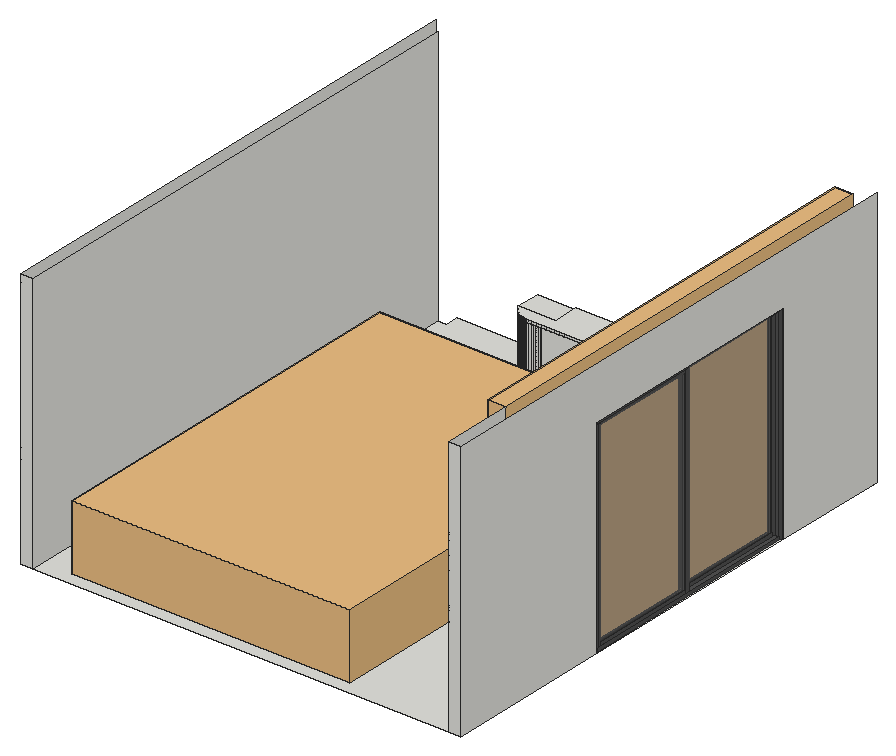
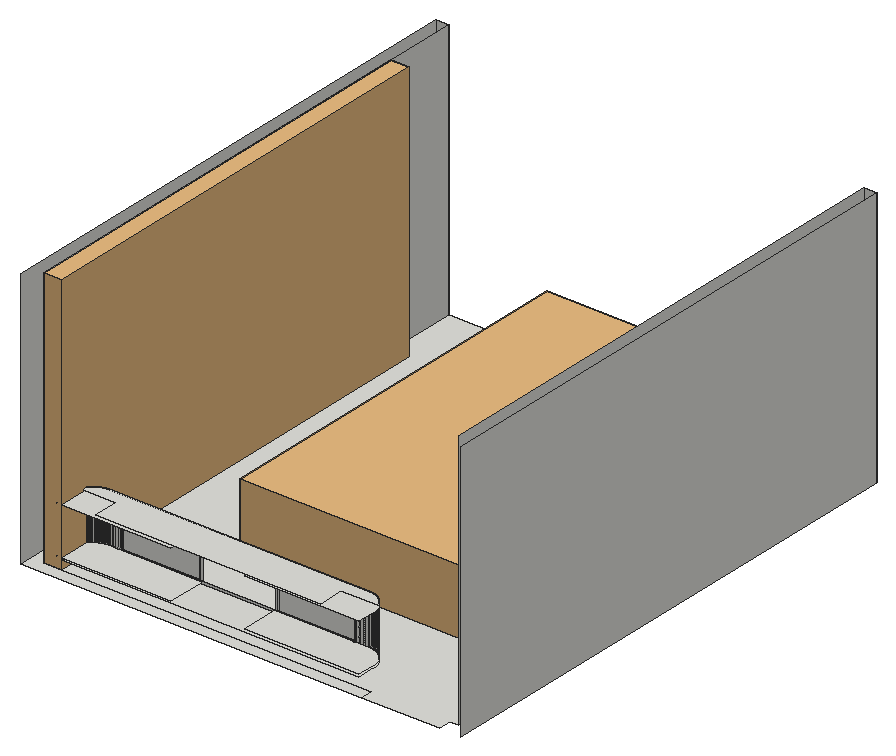
# SketchUp Ruby script. Lengths in inches.
U = 1.inch
M = Sketchup.active_model
def pt(a) = Geom::Point3d.new(a.map { |v| v * U })
def face(e, loops, mat)
  f = e.add_face(loops[0].map { |a| pt(a) })
  loops[1..].each { |l| e.add_face(l.map { |a| pt(a) }).erase! }
  f.material = f.back_material = mat if mat
  f
end
# faces: each face lists its corners as indices into pts; further lists are holes
def faces(e, pts, list, mat = nil) = list.each { |f| face(e, (f[0].is_a?(Array) ? f : [f]).map { |l| l.map { |i| pts[i] } }, mat) }
# xy, xz, yz: faces in a plane at the given z, y or x. An outline is a flat list of corners, or four numbers for a rectangle; further outlines are holes
def ring(l) = l.size == 4 ? [[l[0], l[1]], [l[2], l[1]], [l[2], l[3]], [l[0], l[3]]] : l.each_slice(2).to_a
def flat(e, list, mat, &to3) = list.each { |f| face(e, (f[0].is_a?(Array) ? f : [f]).map { |l| ring(l).map { |u, v| to3.(u, v) } }, mat) }
def xy(e, z, list, mat = nil) = flat(e, list, mat) { |x, y| [x, y, z] }
def xz(e, y, list, mat = nil) = flat(e, list, mat) { |x, z| [x, y, z] }
def yz(e, x, list, mat = nil) = flat(e, list, mat) { |y, z| [x, y, z] }
def lines(e, pts, list) = list.each { |a, b| e.add_line(pt(pts[a]), pt(pts[b])) }
# prism: a flat outline (further loops are holes) pulled along v
def prism(e, loops, v, mat = nil)
  f = face(e, loops, mat); d = Geom::Vector3d.new(v.map { |x| x * U })
  f.pushpull(f.normal.samedirection?(d) ? d.length : -d.length)
end
def box(e, o, s, mat = nil) = prism(e, [[o, [o[0] + s[0], o[1], o[2]], [o[0] + s[0], o[1] + s[1], o[2]], [o[0], o[1] + s[1], o[2]]]], [0, 0, s[2]], mat)
def at(x, y, z, deg = 0) = Geom::Transformation.translation(pt([x, y, z])) * Geom::Transformation.rotation(ORIGIN, Z_AXIS, deg.degrees)
def axes(o, x, y, z) = Geom::Transformation.new([*x, 0, *y, 0, *z, 0, *pt(o).to_a, 1])
def part(name) = M.definitions.add(name)
# library, detail: a bought-in or finely detailed component or shape, given as its bounding box
def library(name, o, s) = part(name).tap { |d| box(d.entities, o, s) }
def detail(e, o, s) = box(e.add_group.entities, o, s)
def put(e, d, t, mat = nil) = e.add_instance(d, t).tap { |i| i.material = mat if mat }
def group(e, t, mat = nil) = e.add_group.tap { |g| g.transformation = t; g.material = mat if mat }.entities
root = M.entities
M.materials.add("[0049_Beige]").color = [245, 245, 220]
M.materials.add("[0135_DarkGray]").color = [81, 81, 81]
M.materials.add("[0136_Charcoal]").color = [35, 35, 35]
M.materials.add("[Aluminum]").color = [179, 179, 179]
M.materials.add("[Translucent Glass Gray]").color = [128, 128, 128]
M.materials["[Translucent Glass Gray]"].alpha = 0.15
c1 = library("Sofa+Set+3+(1)",[-143.38,0,0],[143.38,111.7,30.22])
c2 = part("PENTEK_RP Fineline 50S_Sliding_DoorCase_E1")
box(c2.entities,[0,0,0],[1.51,3.66,99.27],"[0135_DarkGray]")
c3 = part("PENTEK_RP Fineline 50S_SlidingDooe_Case_E2")
box(c3.entities,[0,0,0],[96.25,3.66,1.51],"[0135_DarkGray]")
c4 = part("pentek_RP Fineline 50S_SlidingDoor_Case")
put(c4.entities,c2,at(97.76,0,0))
put(c4.entities,c3,at(1.51,0,0))
put(c4.entities,c2,at(0,0,0))
put(c4.entities,c3,at(1.51,0,97.76))
c5 = part("PENTEK_RP Fineline 50S_SlidingDoor_Glass")
box(c5.entities,[0,0,0],[46.58,0.16,94.39],"[Translucent Glass Gray]")
c6 = part("PENTEK_RP Fineline 50S_SlidingDoor_GlazingBead")
box(c6.entities,[0,0,0],[45.47,0.59,0.56],"[0135_DarkGray]")
c7 = part("PENTEK_RP Fineline 50S_SlidingDoor_GlazingBead_2")
box(c7.entities,[0,0,0],[0.56,0.59,94.39],"[0135_DarkGray]")
c8 = part("PENTEK_RP Fineline 50S_SlidingDoor_Leaf_E1")
xy(c8.entities,0,[[0,0,0.93,1.97],[0.93,1.57,1.49,1.97]],"[0135_DarkGray]")
xy(c8.entities,96.25,[[0,0,0.93,0,0.93,1.57,1.49,1.57,1.49,1.97,0,1.97]],"[0135_DarkGray]")
xz(c8.entities,0,[[0,0,0.93,96.25]],"[0135_DarkGray]")
xz(c8.entities,1.57,[[0.93,0,1.49,95.32],[0.93,95.32,1.49,96.25]],"[0135_DarkGray]")
xz(c8.entities,1.97,[[0,0,1.49,96.25]],"[0135_DarkGray]")
yz(c8.entities,0,[[0,0,1.97,96.25]],"[0135_DarkGray]")
yz(c8.entities,0.93,[[0,0,1.57,0.93],[0,0.93,1.57,95.32],[0,95.32,1.57,96.25]],"[0135_DarkGray]")
yz(c8.entities,1.49,[[1.57,0,1.97,95.32],[1.57,95.32,1.97,96.25]],"[0135_DarkGray]")
c9 = part("PENTEK_RP Fineline 50S_SlidingDoor_Leaf_E2")
xy(c9.entities,0,[[0,0,0,1.57,0.56,1.57,0.56,1.97,46.02,1.97,46.02,1.57,46.58,1.57,46.58,0]],"[0135_DarkGray]")
xy(c9.entities,0.93,[[0,0,46.58,1.57]],"[0135_DarkGray]")
xy(c9.entities,1.49,[[0.56,1.57,46.02,1.97]],"[0135_DarkGray]")
xz(c9.entities,0,[[0,0,46.58,0.93]],"[0135_DarkGray]")
xz(c9.entities,1.57,[[0,0,0.56,0.93],[46.02,0,46.58,0.93],[0.56,0.93,46.02,1.49]],"[0135_DarkGray]")
xz(c9.entities,1.97,[[0.56,0,46.02,1.49]],"[0135_DarkGray]")
yz(c9.entities,0,[[0,0,1.57,0.93]],"[0135_DarkGray]")
yz(c9.entities,0.56,[[1.57,0,1.97,0.93],[1.57,0.93,1.97,1.49]],"[0135_DarkGray]")
yz(c9.entities,46.02,[[1.57,0,1.97,0.93],[1.57,0.93,1.97,1.49]],"[0135_DarkGray]")
yz(c9.entities,46.58,[[0,0,1.57,0.93]],"[0135_DarkGray]")
c10 = part("PENTEK_RP Fineline 50S_SlidingDoor_Leaf2")
put(c10.entities,c5,at(1.49,1.42,0.93))
put(c10.entities,c6,at(1.49,0,94.77))
put(c10.entities,c7,at(46.96,0,0.93))
put(c10.entities,c5,at(1.49,0.59,0.93))
put(c10.entities,c7,at(0.93,0,0.93))
put(c10.entities,c8,at(0,0,0))
put(c10.entities,c8,axes([48.44,0,0],[-1,0,0],[0,1,0],[0,0,1]))
put(c10.entities,c6,at(1.49,0,0.93))
put(c10.entities,c9,axes([0.93,0,96.25],[1,0,0],[0,1,0],[0,0,-1]))
put(c10.entities,c9,at(0.93,0,0))
c11 = part("PENTEK_RP Fineline S_SlidingDoor_Leaf1")
put(c11.entities,c7,at(0.93,0,0.93))
put(c11.entities,c7,at(46.96,0,0.93))
put(c11.entities,c5,at(1.49,1.42,0.93))
put(c11.entities,c6,at(1.49,0,0.93))
put(c11.entities,c5,at(1.49,0.59,0.93))
put(c11.entities,c8,at(0,0,0))
put(c11.entities,c8,axes([48.44,0,0],[-1,0,0],[0,1,0],[0,0,1]))
put(c11.entities,c9,axes([0.93,0,96.25],[1,0,0],[0,1,0],[0,0,-1]))
put(c11.entities,c9,at(0.93,0,0))
put(c11.entities,c6,at(1.49,0,94.77))
c12 = library("Garniza_zaclona\#1",[1.52,0,0],[127.96,8.15,78.72])
c13 = part("Group\#18")
xy(c13.entities,0,[[0,0,0.875,0.875],[9.8125,0,10.6875,0.875]])
xy(c13.entities,1,[[0.875,0,9.8125,0.875]])
xy(c13.entities,2,[[0,0,10.6875,0.875]],"[Aluminum]")
xz(c13.entities,0,[[9.8125,0,10.6875,0,10.6875,2,0.875,2,0.875,1,9.8125,1]])
xz(c13.entities,0,[[0,0,0.875,2]],"[Aluminum]")
xz(c13.entities,0.875,[[0,0,0,2,10.6875,2,10.6875,0,9.8125,0,9.8125,1,0.875,1,0.875,0]],"[Aluminum]")
yz(c13.entities,0,[[0,0,0.875,2]],"[Aluminum]")
yz(c13.entities,0.875,[[0,0,0.875,1]])
yz(c13.entities,9.8125,[[0,0,0.875,1]])
yz(c13.entities,10.6875,[[0,0,0.875,1],[0,1,0.875,2]],"[Aluminum]")
xy(root,-64.65,[[468.52,698.04,660.52,698.04,660.52,776.04,666.52,776.04,666.52,884.48,660.52,884.48,660.52,932.04,508.52,932.04,508.52,938.04,472.52,938.04,472.52,932.04,468.52,932.04],[660.52,698.04,666.52,776.04],[660.52,884.48,666.52,884.48,666.52,938.04,508.52,938.04,508.52,932.04,660.52,932.04]])
xy(root,-60.65,[[524.13,914.04,523.74,914.07,523.35,914.11,522.96,914.16,522.57,914.23,522.1875,914.3125,521.81,914.41,521.43,914.53,521.06,914.65,520.69,914.8,520.33,914.95,519.98,915.125,519.63,915.3125,519.3,915.51,518.97,915.72,518.64,915.95,518.33,916.18,518.03,916.43,517.73,916.69,517.45,916.97,517.18,917.25,516.92,917.54,516.67,917.85,516.43,918.16,516.21,918.48,515.99,918.8125,515.8,919.15,515.61,919.5,515.44,919.85,515.28,920.21,515.14,920.57,515.01,920.95,514.9,921.32,514.8,921.7,514.71,922.09,514.64,922.47,514.59,922.86,514.55,923.25,514.53,923.64,514.52,924.04,514.52,932.04,654.52,932.04,654.52,924.04,654.51,923.64,654.49,923.25,654.45,922.86,654.4,922.47,654.33,922.09,654.24,921.7,654.15,921.32,654.03,920.95,653.9,920.57,653.76,920.21,653.6,919.85,653.43,919.5,653.25,919.15,653.05,918.8125,652.84,918.48,652.61,918.16,652.375,917.85,652.125,917.54,651.86,917.25,651.59,916.97,651.31,916.69,651.02,916.43,650.71,916.18,650.4,915.95,650.08,915.72,649.75,915.51,649.41,915.3125,649.0625,915.125,648.71,914.95,648.35,914.8,647.98,914.65,647.24,914.41,646.86,914.3125,646.47,914.23,646.09,914.16,645.7,914.11,645.31,914.07,644.91,914.04]])
xy(root,-59.65,[[524.52,914.04,523.35,914.11,522.96,914.16,522.57,914.23,522.1875,914.3125,521.81,914.41,521.43,914.53,521.06,914.65,520.69,914.8,520.33,914.95,519.98,915.125,519.63,915.3125,519.3,915.51,518.97,915.72,518.64,915.95,518.33,916.18,518.03,916.43,517.73,916.69,517.45,916.97,517.18,917.25,516.92,917.54,516.67,917.85,516.43,918.16,516.21,918.48,515.99,918.8125,515.8,919.15,515.61,919.5,515.44,919.85,515.28,920.21,515.14,920.57,515.01,920.95,514.9,921.32,514.8,921.7,514.71,922.09,514.64,922.47,514.59,922.86,514.55,923.25,514.53,923.64,514.52,924.04,514.52,932.04,567.52,932.04,567.52,914.04,566.52,914.04,566.52,914.24,530.52,914.24,530.52,914.04],[524.13,914.04,523.74,914.07,523.35,914.11,524.52,914.04],[530.52,914.04,566.52,914.24],[601.52,914.04,601.52,932.04,654.52,932.04,654.52,924.04,654.51,923.64,654.49,923.25,654.45,922.86,654.4,922.47,654.33,922.09,654.24,921.7,654.15,921.32,654.03,920.95,653.9,920.57,653.76,920.21,653.6,919.85,653.43,919.5,653.25,919.15,653.05,918.8125,652.94,918.65,652.84,918.48,652.61,918.16,652.375,917.85,652.25,917.69,652.125,917.54,651.86,917.25,651.59,916.97,651.31,916.69,651.02,916.43,650.71,916.18,650.4,915.95,650.08,915.72,649.75,915.51,649.41,915.3125,649.0625,915.125,648.71,914.95,648.35,914.8,647.98,914.65,647.24,914.41,646.86,914.3125,646.47,914.23,646.09,914.16,645.7,914.11,645.31,914.07,644.91,914.04,638.52,914.04,638.52,914.24,602.52,914.24,602.52,914.04],[602.52,914.04,638.52,914.24]])
xy(root,-59.45,[[530.72,914.04,566.32,914.24],[602.72,914.04,638.32,914.24]])
xy(root,-37.85,[[530.72,914.04,566.32,914.24],[602.72,914.04,638.32,914.24]])
xy(root,-37.65,[[524.52,914.04,523.35,914.11,522.96,914.16,522.57,914.23,522.1875,914.3125,521.81,914.41,521.43,914.53,521.06,914.65,520.69,914.8,520.33,914.95,519.98,915.125,519.63,915.3125,519.3,915.51,518.97,915.72,518.64,915.95,518.33,916.18,518.03,916.43,517.73,916.69,517.45,916.97,517.18,917.25,516.92,917.54,516.67,917.85,516.43,918.16,516.21,918.48,515.99,918.8125,515.8,919.15,515.61,919.5,515.44,919.85,515.28,920.21,515.14,920.57,515.01,920.95,514.9,921.32,514.8,921.7,514.71,922.09,514.64,922.47,514.59,922.86,514.55,923.25,514.53,923.64,514.52,924.04,514.52,932.04,567.52,932.04,567.52,914.04,566.52,914.04,566.52,914.24,530.52,914.24,530.52,914.04],[524.13,914.04,523.74,914.07,523.35,914.11,524.52,914.04],[530.52,914.04,566.52,914.24],[601.52,914.04,601.52,932.04,654.52,932.04,654.52,924.04,654.51,923.64,654.49,923.25,654.45,922.86,654.4,922.47,654.33,922.09,654.24,921.7,654.15,921.32,654.03,920.95,653.9,920.57,653.76,920.21,653.6,919.85,653.43,919.5,653.25,919.15,653.05,918.8125,652.94,918.65,652.84,918.48,652.61,918.16,652.375,917.85,652.25,917.69,652.125,917.54,651.86,917.25,651.59,916.97,651.31,916.69,651.02,916.43,650.71,916.18,650.4,915.95,650.08,915.72,649.75,915.51,649.41,915.3125,649.0625,915.125,648.71,914.95,648.35,914.8,647.98,914.65,647.24,914.41,646.86,914.3125,646.47,914.23,646.09,914.16,645.7,914.11,645.31,914.07,644.91,914.04,638.52,914.04,638.52,914.24,602.52,914.24,602.52,914.04],[602.52,914.04,638.52,914.24]])
xy(root,-36.65,[[524.13,914.04,644.91,914.04,645.31,914.07,645.7,914.11,646.09,914.16,646.47,914.23,646.86,914.3125,647.24,914.41,647.98,914.65,648.35,914.8,648.71,914.95,649.0625,915.125,649.41,915.3125,649.75,915.51,650.08,915.72,650.4,915.95,650.71,916.18,651.02,916.43,651.31,916.69,651.59,916.97,651.86,917.25,652.125,917.54,652.375,917.85,652.61,918.16,652.84,918.48,653.05,918.8125,653.25,919.15,653.43,919.5,653.6,919.85,653.68,920.04,636.52,920.04,636.52,932.04,532.52,932.04,532.52,920.04,515.36,920.04,515.44,919.85,515.61,919.5,515.8,919.15,515.99,918.8125,516.21,918.48,516.43,918.16,516.67,917.85,516.92,917.54,517.18,917.25,517.45,916.97,517.73,916.69,518.03,916.43,518.33,916.18,518.64,915.95,518.97,915.72,519.3,915.51,519.63,915.3125,519.98,915.125,520.33,914.95,520.69,914.8,521.06,914.65,521.43,914.53,521.81,914.41,522.1875,914.3125,522.57,914.23,522.96,914.16,523.35,914.11,523.74,914.07]])
xz(root,698.04,[[462.52,-64.65,468.52,55.35],[660.52,-64.65,666.52,55.35]])
xz(root,776.04,[[660.52,-64.65,666.52,31.35]])
xz(root,884.48,[[660.52,-64.65,666.52,31.35]])
xz(root,914.04,[[524.13,-60.65,524.52,-59.65],[524.52,-60.65,530.52,-59.65],[530.52,-60.65,638.52,-59.65],[638.52,-60.65,644.52,-59.65],[644.52,-60.65,644.91,-59.65],
  [524.13,-59.65,524.52,-37.65],[524.52,-59.65,525.72,-37.65],[525.72,-59.65,526.92,-37.65],[526.92,-59.65,528.12,-37.65],[528.12,-59.65,529.32,-37.65],
  [529.32,-59.65,530.52,-37.65],[566.52,-59.65,567.52,-37.65],[601.52,-59.65,602.52,-37.65],[638.52,-59.65,639.52,-37.65],[639.52,-59.65,640.52,-37.65],
  [640.52,-59.65,641.52,-37.65],[641.52,-59.65,642.52,-37.65],[642.52,-59.65,643.52,-37.65],[643.52,-59.65,644.52,-37.65],[644.52,-59.65,644.91,-37.65],
  [530.72,-59.45,566.32,-37.85],[602.72,-59.45,638.32,-37.85],[567.52,-49.15,601.52,-48.15],[524.13,-37.65,524.52,-36.65],[524.52,-37.65,530.52,-36.65],
  [530.52,-37.65,638.52,-36.65],[638.52,-37.65,644.52,-36.65],[644.52,-37.65,644.91,-36.65]])
xz(root,914.24,[[[530.52,-59.65,566.52,-37.65],[530.72,-59.45,566.32,-37.85]],[[602.52,-59.65,638.52,-37.65],[602.72,-59.45,638.32,-37.85]]],"[0136_Charcoal]")
yz(root,462.52,[[698.04,-64.65,938.04,55.35]])
yz(root,468.52,[[698.04,-64.65,932.04,55.35]])
yz(root,530.52,[[914.04,-59.65,914.24,-37.65]])
yz(root,530.72,[[914.04,-59.45,914.24,-37.85]])
yz(root,566.32,[[914.04,-59.45,914.24,-37.85]])
yz(root,566.52,[[914.04,-59.65,914.24,-37.65]])
yz(root,602.52,[[914.04,-59.65,914.24,-37.65]])
yz(root,602.72,[[914.04,-59.45,914.24,-37.85]])
yz(root,638.32,[[914.04,-59.45,914.24,-37.85]])
yz(root,638.52,[[914.04,-59.65,914.24,-37.65]])
yz(root,660.52,[[698.04,-64.65,698.04,55.35,932.04,55.35,932.04,-64.65,884.48,-64.65,884.48,31.35,776.04,31.35,776.04,-64.65]])
yz(root,666.52,[[698.04,-64.65,776.04,-64.65,776.04,31.35,884.48,31.35,884.48,-64.65,938.04,-64.65,938.04,55.35,698.04,55.35]])
p = [[524.13,914.04,-60.65],[524.13,914.04,-59.65],[523.74,914.07,-59.65],[523.74,914.07,-60.65],[645.31,914.07,-60.65],[645.31,914.07,-59.65],
  [644.91,914.04,-59.65],[644.91,914.04,-60.65],[523.35,914.11,-60.65],[523.35,914.11,-59.65],[522.96,914.16,-59.65],[522.96,914.16,-60.65],
  [645.7,914.11,-60.65],[645.7,914.11,-59.65],[646.09,914.16,-60.65],[646.09,914.16,-59.65],[522.57,914.23,-60.65],[522.57,914.23,-59.65],
  [522.1875,914.3125,-59.65],[522.1875,914.3125,-60.65],[646.47,914.23,-60.65],[646.47,914.23,-59.65],[646.86,914.3125,-60.65],[646.86,914.3125,-59.65],
  [521.81,914.41,-59.65],[521.81,914.41,-60.65],[647.24,914.41,-60.65],[647.24,914.41,-59.65],[521.43,914.53,-59.65],[521.43,914.53,-60.65],
  [647.61,914.53,-60.65],[647.61,914.53,-59.65],[521.06,914.65,-59.65],[521.06,914.65,-60.65],[647.98,914.65,-60.65],[647.98,914.65,-59.65],
  [520.69,914.8,-59.65],[520.69,914.8,-60.65],[648.35,914.8,-60.65],[648.35,914.8,-59.65],[520.33,914.95,-59.65],[520.33,914.95,-60.65],
  [648.71,914.95,-60.65],[648.71,914.95,-59.65],[519.98,915.125,-59.65],[519.98,915.125,-60.65],[649.0625,915.125,-60.65],[649.0625,915.125,-59.65],
  [519.63,915.3125,-59.65],[519.63,915.3125,-60.65],[649.41,915.3125,-60.65],[649.41,915.3125,-59.65],[519.3,915.51,-59.65],[519.3,915.51,-60.65],
  [649.75,915.51,-60.65],[649.75,915.51,-59.65],[518.97,915.72,-59.65],[518.97,915.72,-60.65],[650.08,915.72,-60.65],[650.08,915.72,-59.65],
  [518.64,915.95,-59.65],[518.64,915.95,-60.65],[650.4,915.95,-60.65],[650.4,915.95,-59.65],[518.33,916.18,-59.65],[518.33,916.18,-60.65],
  [650.71,916.18,-60.65],[650.71,916.18,-59.65],[518.03,916.43,-59.65],[518.03,916.43,-60.65],[651.02,916.43,-60.65],[651.02,916.43,-59.65],
  [517.73,916.69,-59.65],[517.73,916.69,-60.65],[651.31,916.69,-60.65],[651.31,916.69,-59.65],[517.45,916.97,-59.65],[517.45,916.97,-60.65],
  [651.59,916.97,-60.65],[651.59,916.97,-59.65],[651.45,916.83,-59.65],[517.18,917.25,-59.65],[517.18,917.25,-60.65],[651.86,917.25,-60.65],
  [651.86,917.25,-59.65],[516.92,917.54,-59.65],[516.92,917.54,-60.65],[652.125,917.54,-60.65],[652.125,917.54,-59.65],[516.67,917.85,-59.65],
  [516.67,917.85,-60.65],[652.375,917.85,-60.65],[652.375,917.85,-59.65],[652.25,917.69,-59.65],[516.43,918.16,-59.65],[516.43,918.16,-60.65],
  [652.61,918.16,-60.65],[652.61,918.16,-59.65],[516.21,918.48,-59.65],[516.21,918.48,-60.65],[652.84,918.48,-60.65],[652.84,918.48,-59.65],
  [524.52,914.04,-37.65],[523.35,914.11,-37.65],[524.52,914.04,-59.65],[524.13,914.04,-37.65],[523.74,914.07,-37.65],[645.31,914.07,-37.65],
  [644.91,914.04,-37.65],[522.96,914.16,-37.65],[645.7,914.11,-37.65],[646.09,914.16,-37.65],[522.57,914.23,-37.65],[522.1875,914.3125,-37.65],
  [646.47,914.23,-37.65],[646.86,914.3125,-37.65],[521.81,914.41,-37.65],[647.24,914.41,-37.65],[521.43,914.53,-37.65],[647.61,914.53,-37.65],
  [521.06,914.65,-37.65],[647.98,914.65,-37.65],[520.69,914.8,-37.65],[648.35,914.8,-37.65],[520.33,914.95,-37.65],[648.71,914.95,-37.65],
  [519.98,915.125,-37.65],[649.0625,915.125,-37.65],[519.63,915.3125,-37.65],[649.41,915.3125,-37.65],[519.3,915.51,-37.65],[649.75,915.51,-37.65],
  [518.97,915.72,-37.65],[650.08,915.72,-37.65],[518.64,915.95,-37.65],[650.4,915.95,-37.65],[518.33,916.18,-37.65],[650.71,916.18,-37.65],
  [518.03,916.43,-37.65],[651.02,916.43,-37.65],[517.73,916.69,-37.65],[651.31,916.69,-37.65],[517.45,916.97,-37.65],[651.45,916.83,-37.65],
  [651.59,916.97,-37.65],[517.18,917.25,-37.65],[651.86,917.25,-37.65],[516.92,917.54,-37.65],[652.125,917.54,-37.65],[516.67,917.85,-37.65],
  [652.25,917.69,-37.65],[652.375,917.85,-37.65],[516.43,918.16,-37.65],[652.61,918.16,-37.65],[516.21,918.48,-37.65],[652.84,918.48,-37.65],
  [524.13,914.04,-36.65],[523.74,914.07,-36.65],[645.31,914.07,-36.65],[644.91,914.04,-36.65],[523.35,914.11,-36.65],[522.96,914.16,-36.65],
  [645.7,914.11,-36.65],[646.09,914.16,-36.65],[522.57,914.23,-36.65],[522.1875,914.3125,-36.65],[646.47,914.23,-36.65],[646.86,914.3125,-36.65],
  [521.81,914.41,-36.65],[647.24,914.41,-36.65],[521.43,914.53,-36.65],[647.61,914.53,-36.65],[521.06,914.65,-36.65],[647.98,914.65,-36.65],
  [520.69,914.8,-36.65],[648.35,914.8,-36.65],[520.33,914.95,-36.65],[648.71,914.95,-36.65],[519.98,915.125,-36.65],[649.0625,915.125,-36.65],
  [519.63,915.3125,-36.65],[649.41,915.3125,-36.65],[519.3,915.51,-36.65],[649.75,915.51,-36.65],[518.97,915.72,-36.65],[650.08,915.72,-36.65],
  [518.64,915.95,-36.65],[650.4,915.95,-36.65],[518.33,916.18,-36.65],[650.71,916.18,-36.65],[518.03,916.43,-36.65],[651.02,916.43,-36.65],
  [517.73,916.69,-36.65],[651.31,916.69,-36.65],[517.45,916.97,-36.65],[651.59,916.97,-36.65],[517.18,917.25,-36.65],[651.86,917.25,-36.65],
  [516.92,917.54,-36.65],[652.125,917.54,-36.65],[516.67,917.85,-36.65],[652.375,917.85,-36.65],[516.43,918.16,-36.65],[652.61,918.16,-36.65]]
faces(root,p,[[0,1,2,3],[4,5,6,7],[8,9,10,11],[3,2,9,8],[12,13,5,4],[14,15,13,12],[16,17,18,19],[11,10,17,16],
  [20,21,15,14],[22,23,21,20],[19,18,24,25],[26,27,23,22],[25,24,28,29],[30,31,27,26],[29,28,32,33],[34,35,31,30],
  [33,32,36,37],[38,39,35,34],[37,36,40,41],[42,43,39,38],[41,40,44,45],[46,47,43,42],[45,44,48,49],[50,51,47,46],
  [49,48,52,53],[54,55,51,50],[53,52,56,57],[58,59,55,54],[57,56,60,61],[62,63,59,58],[61,60,64,65],[66,67,63,62],
  [65,64,68,69],[70,71,67,66],[69,68,72,73],[74,75,71,70],[73,72,76,77],[78,79,80,75,74],[77,76,81,82],[83,84,79,78],
  [82,81,85,86],[87,88,84,83],[86,85,89,90],[91,92,93,88,87],[90,89,94,95],[96,97,92,91],[95,94,98,99],[100,101,97,96],
  [102,103,9,104],[1,105,106,2],[5,107,108,6],[9,103,109,10],[2,106,103,9],[13,110,107,5],[15,111,110,13],[17,112,113,18],
  [10,109,112,17],[21,114,111,15],[23,115,114,21],[18,113,116,24],[27,117,115,23],[24,116,118,28],[31,119,117,27],[28,118,120,32],
  [35,121,119,31],[32,120,122,36],[39,123,121,35],[36,122,124,40],[43,125,123,39],[40,124,126,44],[47,127,125,43],[44,126,128,48],
  [51,129,127,47],[48,128,130,52],[55,131,129,51],[52,130,132,56],[59,133,131,55],[56,132,134,60],[63,135,133,59],[60,134,136,64],
  [67,137,135,63],[64,136,138,68],[71,139,137,67],[68,138,140,72],[75,141,139,71],[72,140,142,76],[75,80,143,141],[144,143,80,79],
  [76,142,145,81],[84,146,144,79],[81,145,147,85],[88,148,146,84],[85,147,149,89],[88,93,150,148],[151,150,93,92],[89,149,152,94],
  [97,153,151,92],[94,152,154,98],[101,155,153,97],[156,157,106,105],[158,159,108,107],[160,161,109,103],[157,160,103,106],[162,158,107,110],
  [163,162,110,111],[164,165,113,112],[161,164,112,109],[166,163,111,114],[167,166,114,115],[165,168,116,113],[169,167,115,117],[168,170,118,116],
  [171,169,117,119],[170,172,120,118],[173,171,119,121],[172,174,122,120],[175,173,121,123],[174,176,124,122],[177,175,123,125],[176,178,126,124],
  [179,177,125,127],[178,180,128,126],[181,179,127,129],[180,182,130,128],[183,181,129,131],[182,184,132,130],[185,183,131,133],[184,186,134,132],
  [187,185,133,135],[186,188,136,134],[189,187,135,137],[188,190,138,136],[191,189,137,139],[190,192,140,138],[193,191,139,141],[192,194,142,140],
  [195,193,141,143,144],[194,196,145,142],[197,195,144,146],[196,198,147,145],[199,197,146,148],[198,200,149,147],[201,199,148,150,151],[200,202,152,149],
  [203,201,151,153]])
put(root,c1,axes([610.02,881.9,-64.65],[0,1.24,0],[-1.15,0,0],[0,0,1]))
g1 = group(root,at(545.17,764.84,-64.65))
xy(g1,0,[[6,6,60.5,66.625]])
xy(g1,2,[[8,6,33.25,6.18],[33.25,6,58.5,18]])
xy(g1,2.2,[[8.2,6,33.05,6.18]])
xy(g1,15.8,[[8.2,6,33.05,6.18]])
xy(g1,16,[[8,6,33.25,6.18],[33.25,6,58.5,18]])
xy(g1,18,[[6,6,60.5,66.625]])
xz(g1,6,[[[6,0,60.5,18],[8,2,58.5,16]],[8.2,2.2,33.05,15.8]])
xz(g1,6.18,[[[8,2,33.25,16],[8.2,2.2,33.05,15.8]]])
xz(g1,18,[[33.25,2,58.5,16]])
xz(g1,66.625,[[6,0,60.5,18]])
yz(g1,6,[[6,0,66.625,18]])
yz(g1,8,[[6,2,6.18,16]])
yz(g1,8.2,[[6,2.2,6.18,15.8]])
yz(g1,33.05,[[6,2.2,6.18,15.8]])
yz(g1,33.25,[[6.18,2,18,16]])
yz(g1,58.5,[[6,2,18,16]])
yz(g1,60.5,[[6,0,66.625,18]])
g2 = group(root,at(661.69,776.04,-64.65))
put(g2,c4,axes([0.39,108.45,0],[0,-1.09241,0],[1,0,0],[0,0,0.96704]))
put(g2,c10,axes([1.97,54.57,1.46],[0,-1.09241,0],[1,0,0],[0,0,0.96704]))
put(g2,c11,axes([0,106.8,1.46],[0,-1.09241,0],[1,0,0],[0,0,0.96704]))
put(root,c12,axes([652.37,934.375,-64.65],[0,-1.5698,0],[1,0,0],[0,0,1.52445]),"[0049_Beige]")
put(root,c13,axes([543.84,914.04,-44.13],[1,0,0],[0,0,1],[0,-1,0]),"[Aluminum]")
put(root,c13,axes([614.9,914.04,-44.13],[1,0,0],[0,0,1],[0,-1,0]),"[Aluminum]")
